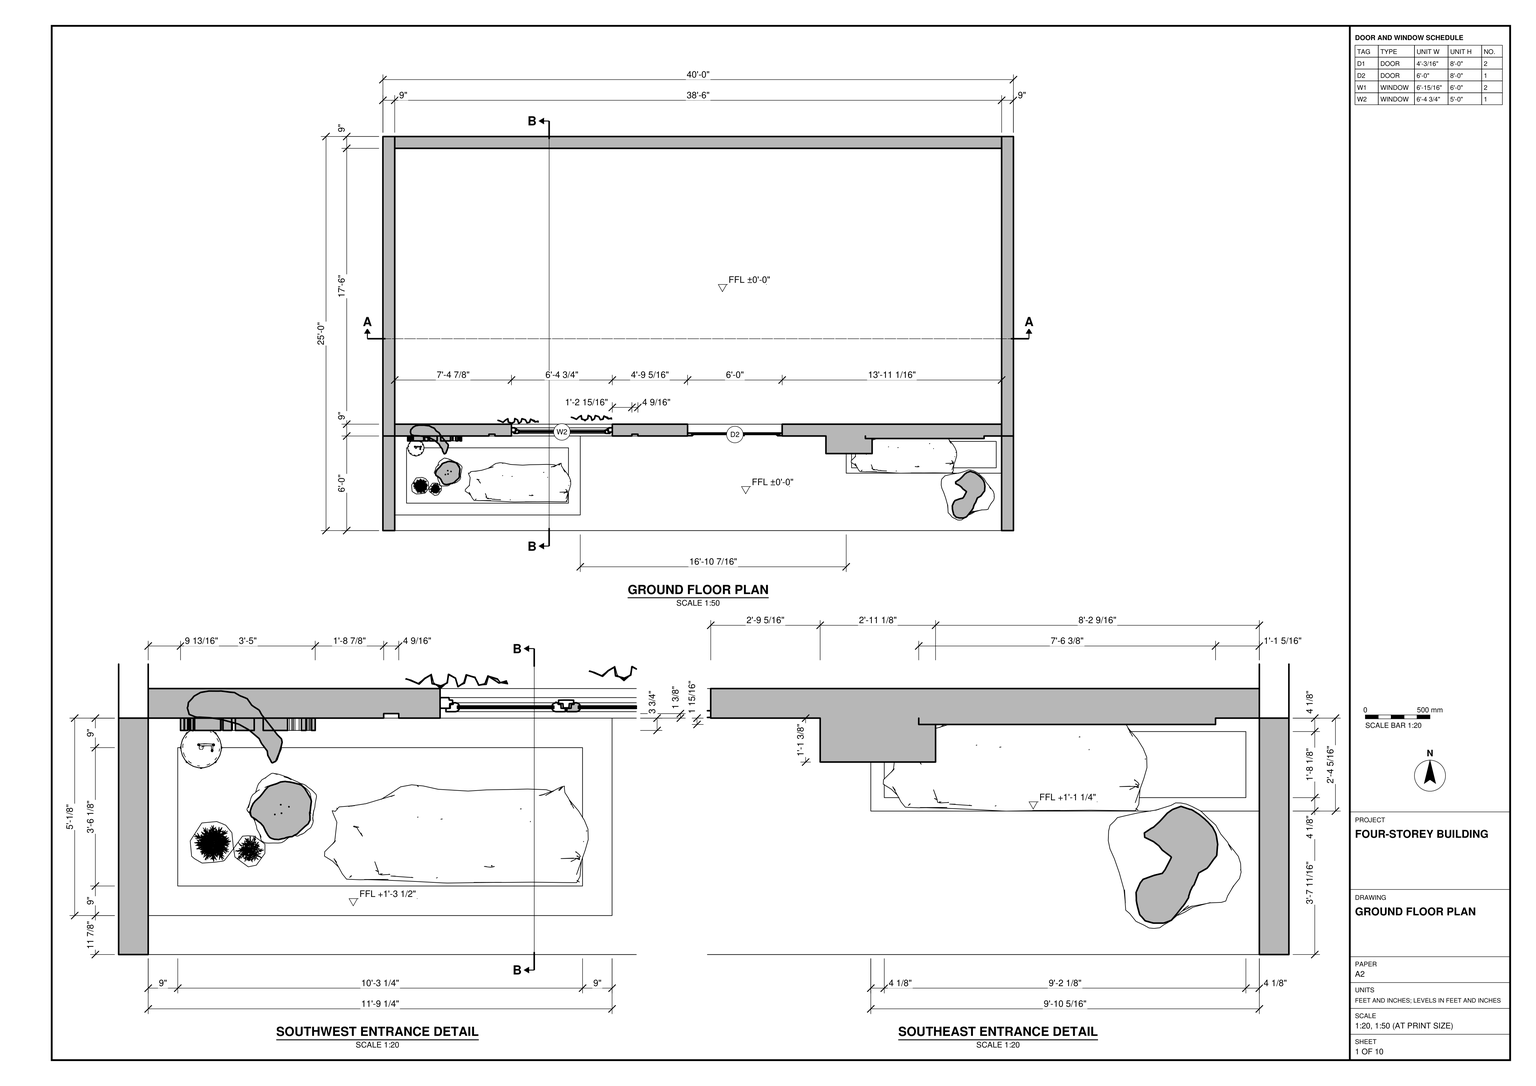
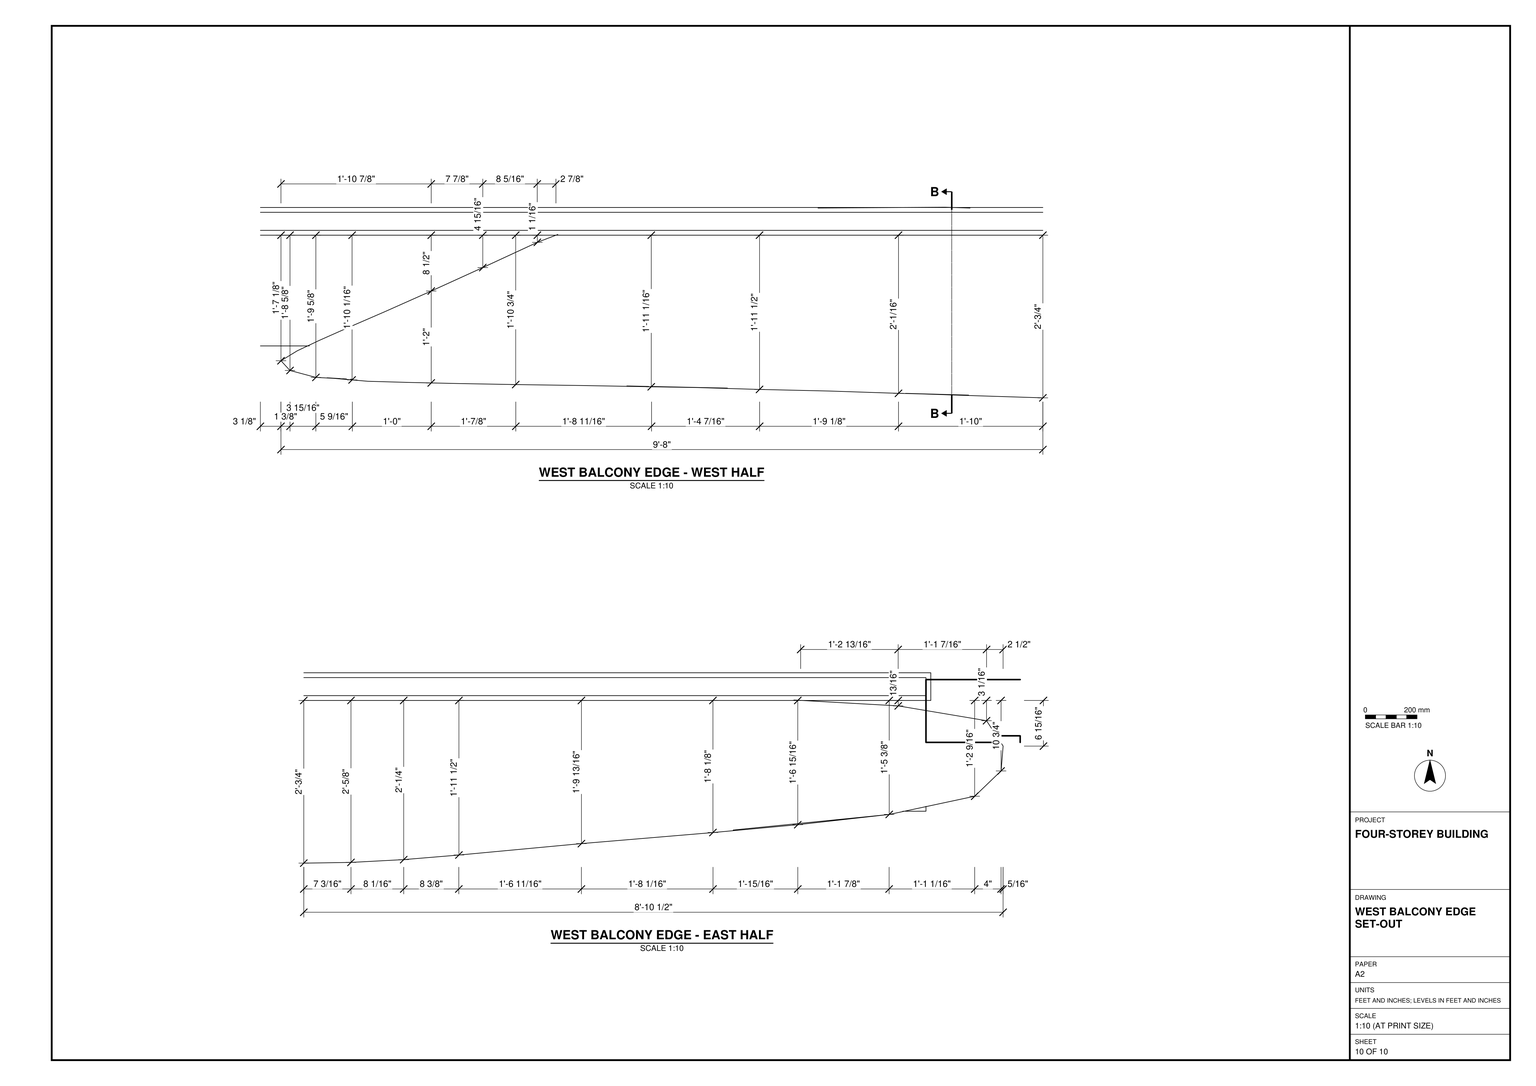
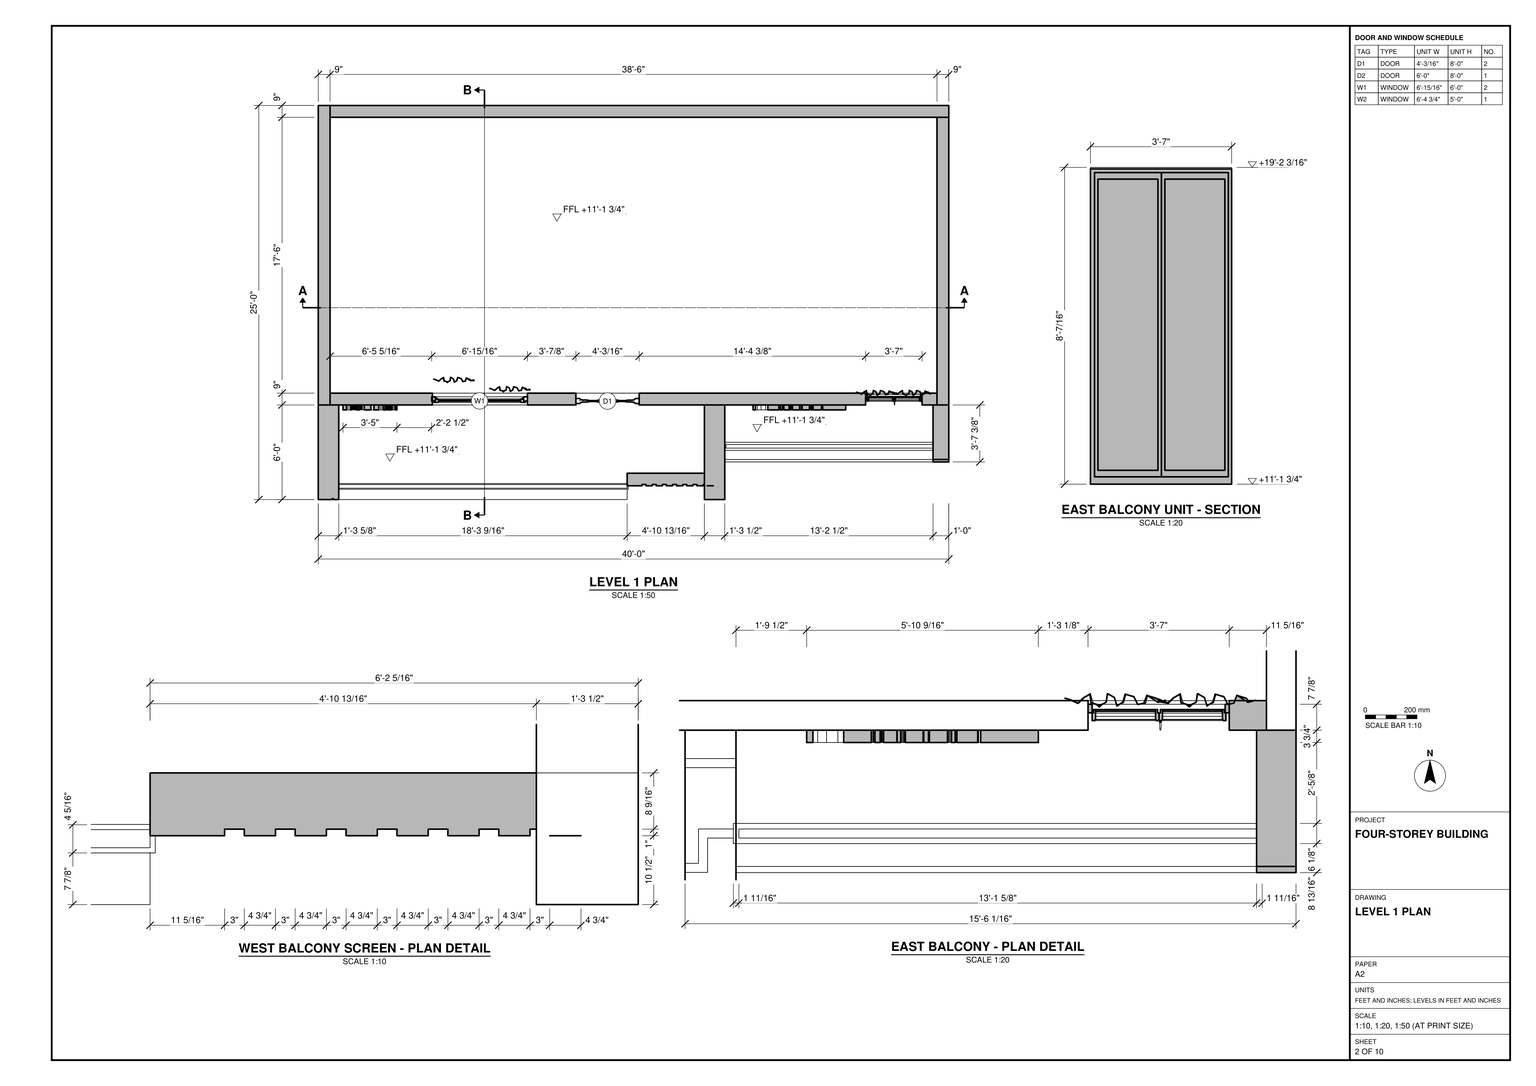
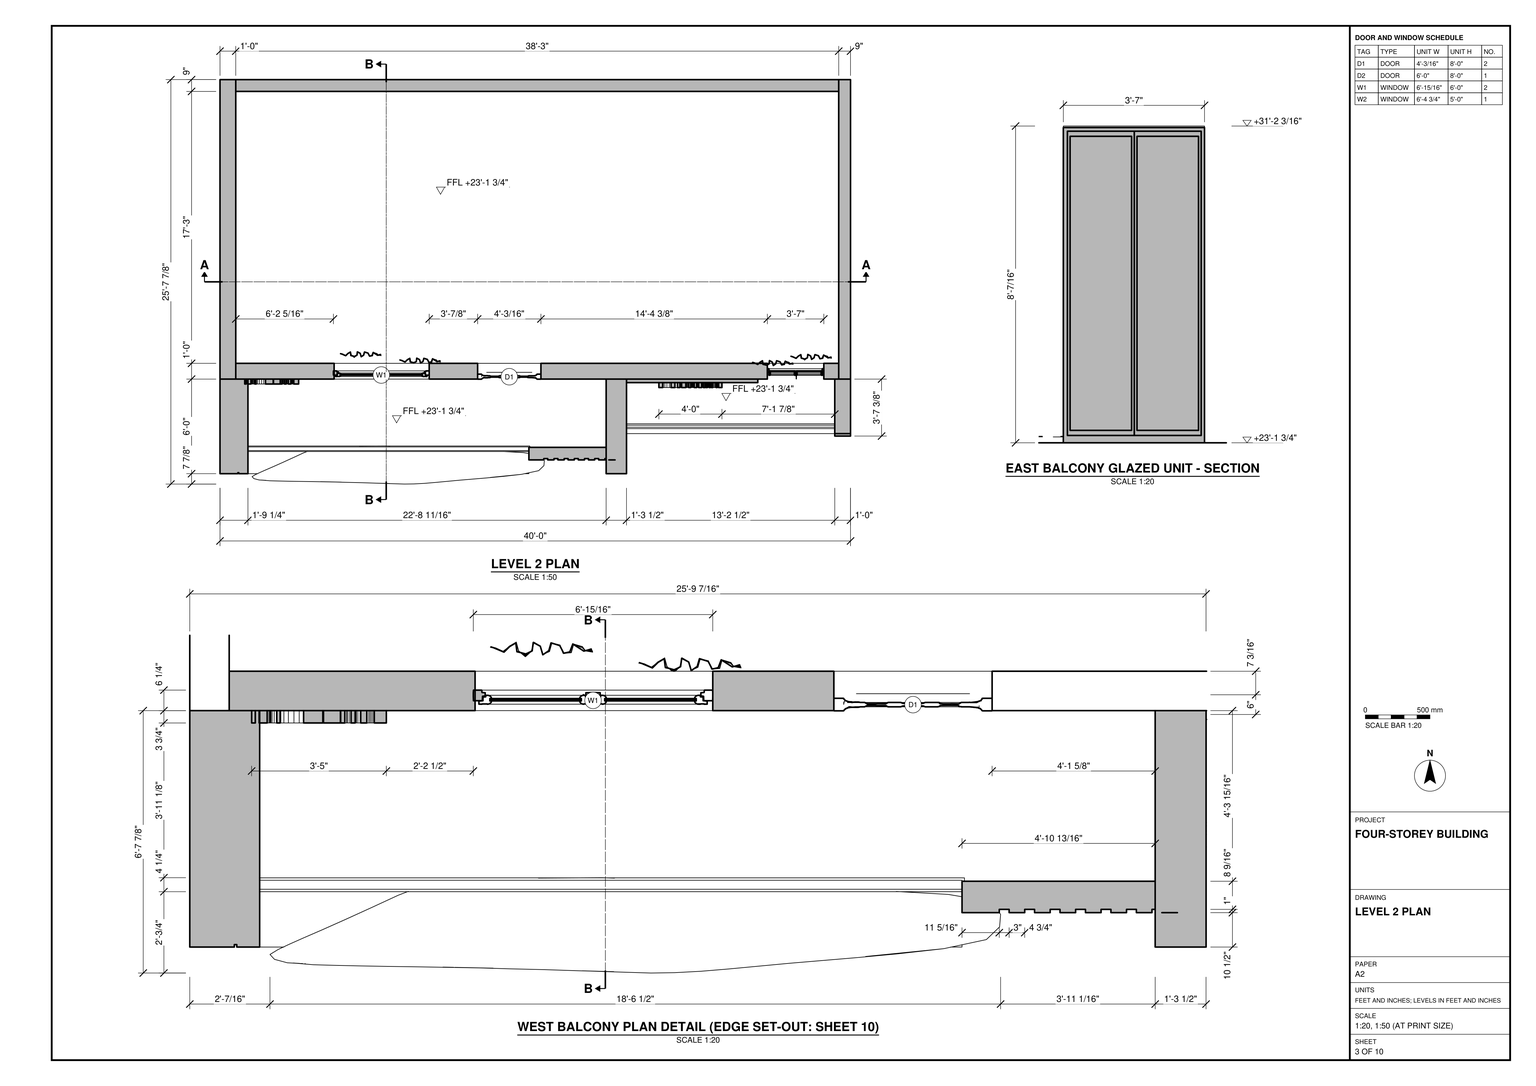
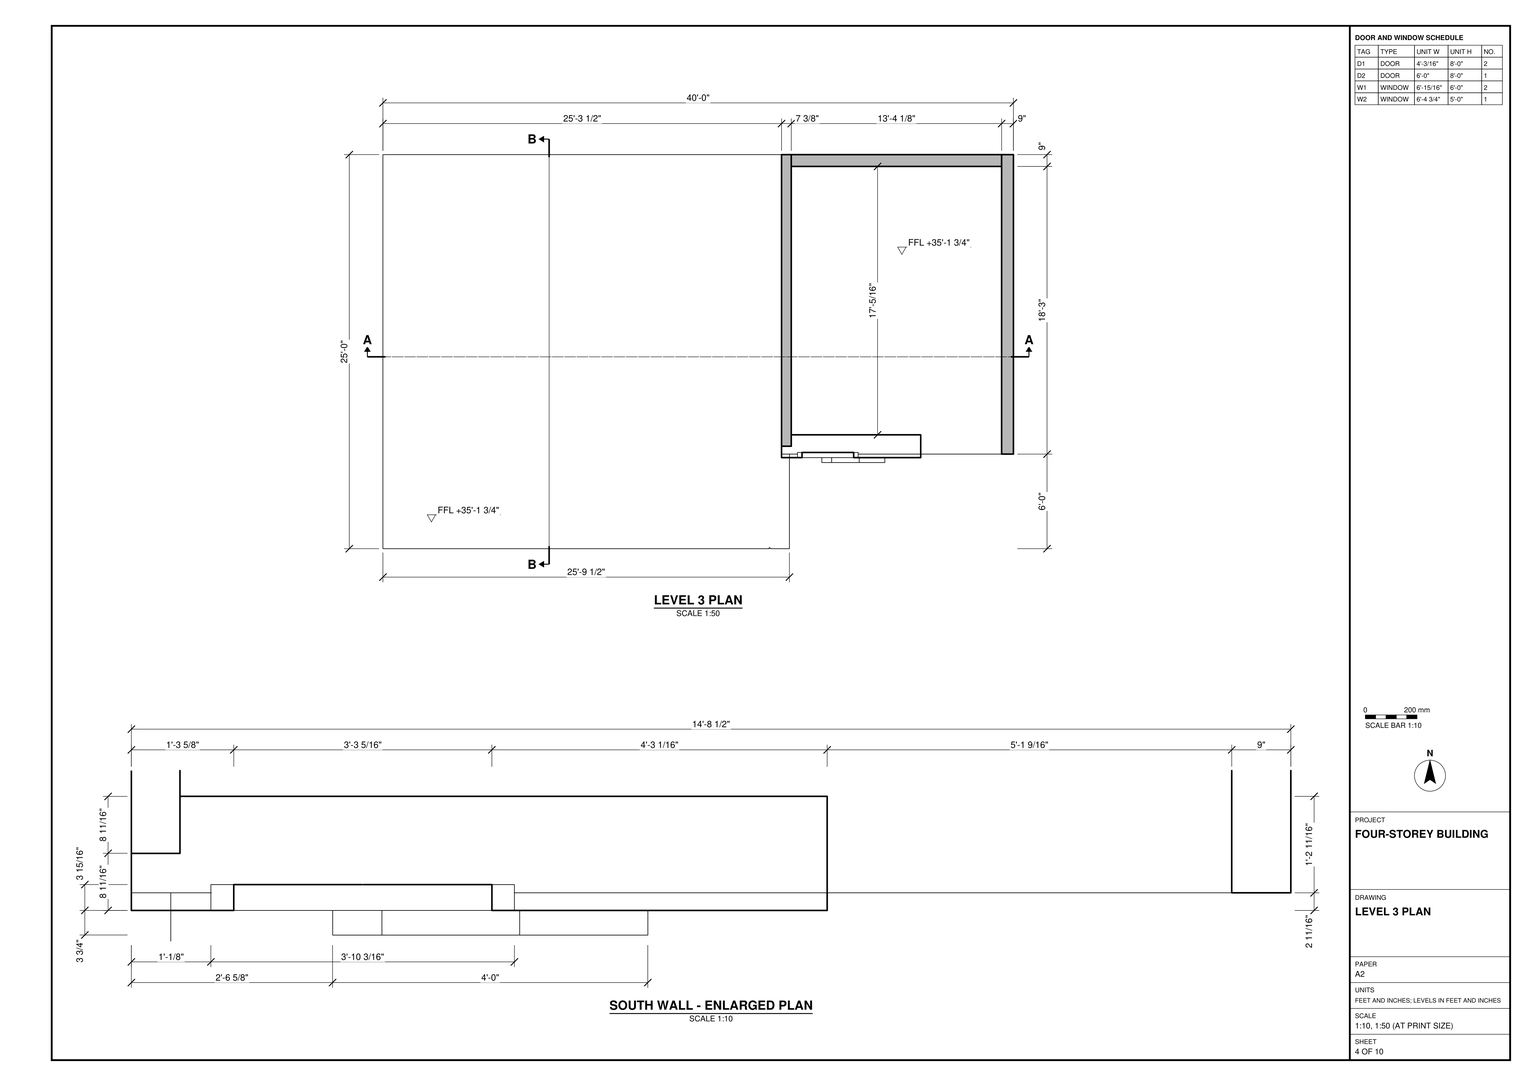
Build the four-storey building in SketchUp using task_files/diagram_01.pdf. Work in feet and inches. The overall model extents are 40'-0" from west to east, 25'-7 7/8" from front to back and 42'-7 3/4" in height. Set the floor levels to ±0'-0", +11'-1 3/4", +23'-1 3/4" and +35'-1 3/4".

Lay out the ground floor with the 9" walls shown in plan. Extend the side walls past the entrance wall to frame the 6'-0" deep entrance area. Place the front window west of the entrance door, and model the raised planting beds at the two ends of the entrance. Above it, distinguish the wider west balcony from the shallower east balcony. Use the enlarged details for the west balcony screen, the shaped balcony edge and the paired glazed panels at the east balcony.

Follow the plans, elevations and sections for the upper walls, floor slabs, openings and roof profile. Include stairs, built-in joinery and main furniture where shown. Keep walls, slabs, roof and each furniture or joinery piece in separate groups or components, and use components for repeated parts. Plants and other loose decorative items may be any suitable library components. Save one SketchUp model as output_files/four_storey_building_with_its_entrance_and_balconies.skp.

# SketchUp Ruby script. Lengths in inches.
U = 1.inch
M = Sketchup.active_model
def pt(a) = Geom::Point3d.new(a.map { |v| v * U })
def face(e, loops, mat)
  f = e.add_face(loops[0].map { |a| pt(a) })
  loops[1..].each { |l| e.add_face(l.map { |a| pt(a) }).erase! }
  f.material = f.back_material = mat if mat
  f
end
# faces: each face lists its corners as indices into pts; further lists are holes
def faces(e, pts, list, mat = nil) = list.each { |f| face(e, (f[0].is_a?(Array) ? f : [f]).map { |l| l.map { |i| pts[i] } }, mat) }
# xy, xz, yz: faces in a plane at the given z, y or x. An outline is a flat list of corners, or four numbers for a rectangle; further outlines are holes
def ring(l) = l.size == 4 ? [[l[0], l[1]], [l[2], l[1]], [l[2], l[3]], [l[0], l[3]]] : l.each_slice(2).to_a
def flat(e, list, mat, &to3) = list.each { |f| face(e, (f[0].is_a?(Array) ? f : [f]).map { |l| ring(l).map { |u, v| to3.(u, v) } }, mat) }
def xy(e, z, list, mat = nil) = flat(e, list, mat) { |x, y| [x, y, z] }
def xz(e, y, list, mat = nil) = flat(e, list, mat) { |x, z| [x, y, z] }
def yz(e, x, list, mat = nil) = flat(e, list, mat) { |y, z| [x, y, z] }
def lines(e, pts, list) = list.each { |a, b| e.add_line(pt(pts[a]), pt(pts[b])) }
# prism: a flat outline (further loops are holes) pulled along v
def prism(e, loops, v, mat = nil)
  f = face(e, loops, mat); d = Geom::Vector3d.new(v.map { |x| x * U })
  f.pushpull(f.normal.samedirection?(d) ? d.length : -d.length)
end
def box(e, o, s, mat = nil) = prism(e, [[o, [o[0] + s[0], o[1], o[2]], [o[0] + s[0], o[1] + s[1], o[2]], [o[0], o[1] + s[1], o[2]]]], [0, 0, s[2]], mat)
def at(x, y, z, deg = 0) = Geom::Transformation.translation(pt([x, y, z])) * Geom::Transformation.rotation(ORIGIN, Z_AXIS, deg.degrees)
def axes(o, x, y, z) = Geom::Transformation.new([*x, 0, *y, 0, *z, 0, *pt(o).to_a, 1])
def part(name) = M.definitions.add(name)
# library, detail: a bought-in or finely detailed component or shape, given as its bounding box
def library(name, o, s) = part(name).tap { |d| box(d.entities, o, s) }
def detail(e, o, s) = box(e.add_group.entities, o, s)
def put(e, d, t, mat = nil) = e.add_instance(d, t).tap { |i| i.material = mat if mat }
def group(e, t, mat = nil) = e.add_group.tap { |g| g.transformation = t; g.material = mat if mat }.entities
root = M.entities
M.materials.add("Emissive").color = [230, 236, 181]
M.materials.add("Marble White SSS 100cm").color = [222, 222, 222]
M.materials.add("[Color H07]").color = [0, 153, 153]
M.materials.add("[Translucent Glass Blue]").color = [100, 149, 237]
M.materials["[Translucent Glass Blue]"].alpha = 0.5
M.materials.add("[Wood Veneer 01]").color = [120, 70, 37]
c1 = library("Curtains 004",[-15.59,-2.26,0],[31.18,4.52,116.91])
c2 = library("Door 243 067",[-20.85,-3,0],[41.7,6,82.46])
c3 = library("Elegant door(double)",[38.88,29.07,0],[76.71,4.33,84.81])
c4 = library("porta_finestra_2ante",[2.73,-0.04,0],[81.59,5.98,96.46])
c5 = library("Window 46-15",[-34.06,-3.13,0],[68.12,6.24,59.06])
c6 = library("Viola hederacea 011",[-26.29,-11.24,-33.88],[55.62,29.03,38.84])
c7 = library("Viola hederacea 004",[-17.97,-14.58,0.39],[33.12,31.94,9.08])
c8 = library("False Aralia 002",[-20.33,-19.19,0],[40.48,38.23,49.87])
c9 = library("Potted Tree 19",[-18.04,-21.3125,0],[43.7,42.65,66.52])
c10 = library("Potted Plants 50-15",[-11.38,-6.89,0],[22.76,13.78,19.62])
c11 = library("Potted Plant 60-25",[-10.7,-10.47,0],[21.2,21.27,47.12])
c12 = library("Potted Flowers 111-27",[-6.96,-10.89,0.07],[14.96,24.75,20.38])
c13 = library("c103.dxf",[0,0,0],[4.7,1.18,0.06])
xy(root,-12,[[0,0,480,300]])
xy(root,0,[[0,0,9,72],[9,0,471,0,471,43.6875,352.6875,43.6875,352.6875,72,303.9375,72,303.9375,81,231.9375,81,231.9375,72,150.25,72,150.25,11.875,9,11.875],[471,0,480,72],[9,11.875,150.25,72],[0,72,9,300],
  [9,72,231.9375,81],[303.9375,72,471,81],[471,72,480,300],[9,81,471,291],[9,291,471,300]])
xy(root,8.19,[[367.29,70.0625,457.66,72]])
xy(root,10.875,[[17.99,20.87,141.26,63.01],[356.79,47.79,466.9,67.9]],"[Wood Veneer 01]")
xy(root,13.25,[[[352.6875,43.6875,471,72],[356.79,47.79,466.9,67.9]]],"[Wood Veneer 01]")
xy(root,15.5,[[[9,11.875,150.25,72],[17.99,20.87,141.26,63.01]]],"[Wood Veneer 01]")
xy(root,17.73,[[80.71,72,194.125,73.375]],"Emissive")
xy(root,22.3125,[[85.29,72,189.54,73.375]],"Emissive")
xy(root,36,[[97.875,72,174.625,81]],"Marble White SSS 100cm")
xy(root,39.07,[[337.27,58.625,346.66,72],[346.66,58.625,346.66,72,367.29,72,367.29,70.0625,372.41,70.0625,372.41,58.625]],"[Wood Veneer 01]")
xy(root,47.25,[[337.27,58.625,346.66,72],[346.66,58.625,372.41,58.625,372.41,70.0625,367.29,70.0625,367.29,72,346.66,72]],"[Wood Veneer 01]")
xy(root,69.27,[[337.27,58.625,346.66,72],[346.66,58.625,346.66,72,367.29,72,367.29,70.0625,372.41,70.0625,372.41,58.625]],"[Wood Veneer 01]")
xy(root,72,[[0,0,9,72],[471,0,480,72]])
xy(root,77.96,[[337.27,58.625,346.66,72],[346.66,58.625,372.41,58.625,372.41,70.0625,367.29,70.0625,367.29,72,346.66,72]],"[Wood Veneer 01]")
xy(root,96,[[231.9375,72,303.9375,81]])
xy(root,96,[[97.875,72,174.625,81]],"Marble White SSS 100cm")
xy(root,105.38,[[367.29,70.0625,457.66,72]],"Marble White SSS 100cm")
xy(root,108.8125,[[85.29,72,189.54,73.375]],"Emissive")
xy(root,113.4,[[80.71,72,194.125,73.375]],"Emissive")
xy(root,113.6875,[[293.96,0,309.47,72],[235.15,10.48,235.15,72,293.96,72,293.96,11.48,292.99,11.48,292.99,10.48,288.24,10.48,288.24,11.48,285.24,11.48,285.24,10.48,280.49,10.48,280.49,11.48,277.49,11.48,277.49,10.48,272.74,10.48,272.74,11.48,269.74,11.48,269.74,10.48,264.99,10.48,264.99,11.48,261.99,11.48,261.99,10.48,257.24,10.48,257.24,11.48,254.24,11.48,254.24,10.48,249.49,10.48,249.49,11.48,246.49,11.48,246.49,10.48]])
xy(root,117.6875,[[0,0,0,72,12.01,72,12.01,12.01,208.33,12.01,208.33,72,235.15,72,235.15,0]])
xy(root,118.875,[[[309.47,28.625,471,72],[318.44,37.6,462.02,63.02]],[471,28.625,480,72],[321.41,40.57,459.05,60.05]],"[Wood Veneer 01]")
xy(root,120,[[293.96,0,309.47,20.04],[[12.01,12.01,208.33,72],[19.9,19.9,200.44,64.11]],[293.96,20.04,309.47,72],[24.62,24.62,195.72,59.39],[471,30.5,480,72],
  [0,72,9,300],[9,72,471,81],[471,72,480,300],[9,81,471,291],[9,291,471,300]])
xy(root,120,[[309.47,30.5,471,72]],"[Wood Veneer 01]")
xy(root,120.3125,[[[318.44,37.6,462.02,63.02],[321.41,40.57,459.05,60.05]]])
xy(root,121.4375,[[[19.9,19.9,200.44,64.11],[24.62,24.62,195.72,59.39]]])
xy(root,128.5625,[[10.72,0,11.47,0.75],[11.47,0,235.15,0.75]])
xy(root,129.3125,[[11.47,0,235.15,0.75]])
xy(root,131.8125,[[309.47,28.625,468,30.5]],"[Wood Veneer 01]")
xy(root,133.75,[[15.6,0,235.15,8.65],[15.6,8.65,235.15,11.41],[15.6,11.41,235.15,11.41,235.15,20.04,309.47,20.04,309.47,30.5,468,30.5,468,39.15,310.35,39.15,310.35,41.91,468,41.91,468,72,459.66,72,459.66,81,416.67,81,416.67,72,244.3125,72,244.3125,81,196.125,81,196.125,72,15.6,72],[468,30.5,480,72],[310.35,39.15,468,41.91],
  [0,72,9,300],[9,72,196.125,81],[244.3125,72,416.67,81],[459.66,72,471,81],[471,72,480,291],
  [9,81,471,291],[9,291,480,300]])
xy(root,157.75,[[86.875,72,159.25,81]])
xy(root,169.75,[[15.6,8.65,235.15,11.41],[310.35,39.15,468,41.91]])
xy(root,169.75,[[[14.81,7.86,235.94,12.2],[15.6,8.65,235.15,11.41]],[[308.66,37.46,469.6875,43.6],[310.35,39.15,468,41.91]]],"[Color H07]")
xy(root,170.3125,[[[14.81,7.86,235.94,12.2],[15.6,8.65,235.15,11.41]],[15.6,8.65,235.15,11.41],[[308.66,37.46,469.6875,43.6],[310.35,39.15,468,41.91]],[310.35,39.15,468,41.91]],"[Color H07]")
xy(root,181.75,[[0,0,10.72,0,10.72,0.75,11.47,0.75,11.47,0,15.6,0,15.6,72,0,72]])
xy(root,229.75,[[86.875,72,159.25,81],[196.125,72,244.3125,81],[416.67,72,459.66,81]])
xy(root,253.75,[[0,0,0,72,21.28,72,21.28,0,14.3125,0,14.3125,0.75,13.5625,0.75,13.5625,0],[0,72,9,300],[9,72,471,81],[471,72,480,291],[9,81,471,291],
  [9,291,480,300]])
xy(root,253.75,[[[21.28,0,21.28,72,480,72,480,30.5,309.47,30.5,309.47,20.04,235.15,20.04,235.15,0],[31.97,10.6875,224.46,61.3125],[322.45,41.96,453.17,60.54]],[35.875,14.6,220.55,57.4],[325.58,45.1,450.03,57.4]],"[Wood Veneer 01]")
xy(root,255.1875,[[[31.97,10.6875,224.46,61.3125],[35.875,14.6,220.55,57.4]],[[322.45,41.96,453.17,60.54],[325.58,45.1,450.03,57.4]]],"[Wood Veneer 01]")
xy(root,256.43,[[21.28,0,235.15,0.75]],"[Wood Veneer 01]")
xy(root,257.18,[[21.28,0,235.15,0.75]],"[Wood Veneer 01]")
xy(root,259.86,[[21.28,0,235.15,0.75]],"[Wood Veneer 01]")
xy(root,260.61,[[21.28,0,235.15,0.75]],"[Wood Veneer 01]")
xy(root,263.29,[[21.28,0,235.15,0.75]],"[Wood Veneer 01]")
xy(root,264.04,[[21.28,0,235.15,0.75]],"[Wood Veneer 01]")
xy(root,266.71,[[21.28,0,235.15,0.75]],"[Wood Veneer 01]")
xy(root,267.46,[[21.28,0,235.15,0.75]],"[Wood Veneer 01]")
xy(root,270.14,[[21.28,0,235.15,0.75]],"[Wood Veneer 01]")
xy(root,270.89,[[21.28,0,235.15,0.75]],"[Wood Veneer 01]")
xy(root,273.57,[[21.28,0,235.15,0.75]],"[Wood Veneer 01]")
xy(root,274.32,[[21.28,0,235.15,0.75]],"[Wood Veneer 01]")
xy(root,277.75,[[21.28,17.6,235.15,20.35],[235.15,20.04,309.47,20.04,309.47,72,244.3125,72,244.3125,84,196.125,84,196.125,72,21.28,72,21.28,20.35,235.15,20.35],[309.47,30.5,480,30.5,480,72,459.66,72,459.66,84,416.67,84,416.67,72,409.41,72,409.41,69.3125,309.47,69.3125,309.47,36.9,468,36.9,468,35.36,309.47,35.36],[309.47,35.36,314.32,36.9],[314.32,35.36,468,36.9],
  [0,72,12,300],[12,72,196.125,84],[244.3125,72,416.67,84],[459.66,72,471,84],[471,72,480,300],
  [12,84,471,291],[12,291,471,300]])
xy(root,277.75,[[21.28,0,235.15,17.6]],"[Wood Veneer 01]")
xy(root,301.75,[[86.875,72,159.25,84]])
xy(root,313.75,[[21.28,17.6,235.15,20.35],[309.47,35.36,468,36.9]])
xy(root,313.75,[[[20.54,16.86,235.89,21.08],[21.28,17.6,235.15,20.35]],[[308.41,34.3,469.06,37.96],[309.47,35.36,468,36.9]]],"[Color H07]")
xy(root,314.3125,[[[20.54,16.86,235.89,21.08],[21.28,17.6,235.15,20.35]],[21.28,17.6,235.15,20.35],[[308.41,34.3,469.06,37.96],[309.47,35.36,468,36.9]],[309.47,35.36,468,36.9]],"[Color H07]")
xy(root,337.75,[[468,28.625,480,30.5],[468,30.5,480,72]])
xy(root,373.75,[[86.875,72,159.25,84],[196.125,72,244.3125,84],[416.67,72,459.66,84]])
xy(root,397.75,[[0,0,12,72],[[21.28,0,21.28,72,293.96,72,293.96,20.04,235.15,20.04,235.15,10.48,246.49,10.48,246.49,11.48,249.49,11.48,249.49,10.48,254.24,10.48,254.24,11.48,257.24,11.48,257.24,10.48,261.99,10.48,261.99,11.48,264.99,11.48,264.99,10.48,269.74,10.48,269.74,11.48,272.74,11.48,272.74,10.48,277.49,10.48,277.49,11.48,280.49,11.48,280.49,10.48,285.24,10.48,285.24,11.48,288.24,11.48,288.24,10.48,292.99,10.48,292.99,11.48,293.96,11.48,293.96,0],[155.72,13.26,230.91,13.26,230.91,69.88,223.53,69.88,223.53,20.57,162.28,20.57,162.28,69.88,155.72,69.88],[40.85,13.44,116.03,13.44,116.03,70.07,108.66,70.07,108.66,20.76,47.41,20.76,47.41,70.07,40.85,70.07]],[293.96,0,309.47,72],[235.15,10.48,246.49,10.48,246.49,11.48,249.49,11.48,249.49,10.48,254.24,10.48,254.24,11.48,257.24,11.48,257.24,10.48,261.99,10.48,261.99,11.48,264.99,11.48,264.99,10.48,269.74,10.48,269.74,11.48,272.74,11.48,272.74,10.48,277.49,10.48,277.49,11.48,280.49,11.48,280.49,10.48,285.24,10.48,285.24,11.48,288.24,11.48,288.24,10.48,292.99,10.48,292.99,11.48,293.96,11.48,293.96,20.04,235.15,20.04],[0,72,12,300],
  [12,84,471,291],[12,291,471,300]])
xy(root,399.9375,[[155.72,13.26,155.72,69.88,162.28,69.88,162.28,20.57,223.53,20.57,223.53,69.88,230.91,69.88,230.91,13.26],[40.85,13.44,40.85,70.07,47.41,70.07,47.41,20.76,108.66,20.76,108.66,70.07,116.03,70.07,116.03,13.44]])
xy(root,403,[[14.3125,0,293.96,0.75],[293.96,0,294.71,0.75]])
xy(root,403.75,[[13.5625,0,293.96,0.75]])
xy(root,421.75,[[0,0,293.96,0,293.96,0.75,294.71,0.75,294.71,0,309.47,0,309.47,69.3125,303.47,69.3125,303.47,300,0,300],[303.47,69.3125,309.47,72],[303.47,72,303.47,78,310.87,78,310.87,86.6875,409.41,86.6875,409.41,72],[409.41,72,471,72,471,291,310.87,291,310.87,86.6875,409.41,86.6875],[471,72,480,300],
  [303.47,78,310.87,300],[310.87,291,471,300]])
xy(root,493.75,[[292.53,57.5625,292.53,300,303.47,300,303.47,69.3125,409.41,69.3125,409.41,78,471,78,471,72,480,72,480,57.5625],[303.47,69.3125,310.87,72],[310.87,69.3125,409.41,72],[303.47,72,310.87,78],[310.87,72,409.41,78],
  [471,72,480,300],[303.47,78,310.87,300],[310.87,78,409.41,86.6875],[310.87,291,471,300]])
xy(root,499.75,[[[292.53,57.5625,480,300],[310.87,78,471,291]]])
xz(root,0,[[0,-12,480,0],[0,0,9,72],[471,0,480,72],[293.96,113.6875,309.47,120],[0,117.6875,235.15,117.6875,235.15,128.5625,10.72,128.5625,10.72,181.75,0,181.75],
  [293.96,120,309.47,397.75],[11.47,129.3125,235.15,129.3125,235.15,133.75,15.6,133.75,15.6,181.75,11.47,181.75],[0,253.75,13.5625,397.75],[14.3125,253.75,21.28,397.75],[0,397.75,13.5625,397.75,13.5625,403.75,293.96,403.75,293.96,421.75,0,421.75],
  [14.3125,397.75,309.47,397.75,309.47,421.75,294.71,421.75,294.71,403,14.3125,403]])
xz(root,0,[[21.28,253.75,235.15,256.43],[21.28,257.18,235.15,259.86],[21.28,260.61,235.15,263.29],[21.28,264.04,235.15,266.71],[21.28,267.46,235.15,270.14],
  [21.28,270.89,235.15,273.57],[21.28,274.32,235.15,277.75]],"[Wood Veneer 01]")
xz(root,0.75,[[10.72,128.5625,235.15,128.5625,235.15,129.3125,11.47,129.3125,11.47,181.75,10.72,181.75],[13.5625,253.75,14.3125,397.75],[13.5625,397.75,14.3125,403],[13.5625,403,294.71,403,294.71,421.75,293.96,421.75,293.96,403.75,13.5625,403.75]])
xz(root,0.75,[[21.28,256.43,235.15,257.18],[21.28,259.86,235.15,260.61],[21.28,263.29,235.15,264.04],[21.28,266.71,235.15,267.46],[21.28,270.14,235.15,270.89],
  [21.28,273.57,235.15,274.32]],"[Wood Veneer 01]")
xz(root,7.86,[[14.81,169.75,235.94,170.3125]],"[Color H07]")
xz(root,8.65,[[15.6,169.75,235.15,170.3125]])
xz(root,8.65,[[15.6,133.75,235.15,169.75]],"[Translucent Glass Blue]")
xz(root,10.48,[[235.15,113.6875,241.74,397.75],[241.74,113.6875,246.49,397.75],[249.49,113.6875,254.24,397.75],[257.24,113.6875,261.99,397.75],[264.99,113.6875,269.74,397.75],
  [272.74,113.6875,277.49,397.75],[280.49,113.6875,285.24,397.75],[288.24,113.6875,292.99,397.75],[295.99,113.6875,300.74,397.75]])
xz(root,10.6875,[[31.97,253.75,224.46,255.1875]],"Emissive")
xz(root,11.41,[[226.5,133.75,235.15,169.75],[15.6,169.75,226.5,170.3125],[226.5,169.75,235.15,170.3125]])
xz(root,11.41,[[15.6,133.75,226.5,169.75]],"[Translucent Glass Blue]")
xz(root,11.48,[[246.49,113.6875,249.49,397.75],[254.24,113.6875,257.24,397.75],[261.99,113.6875,264.99,397.75],[269.74,113.6875,272.74,397.75],[277.49,113.6875,280.49,397.75],
  [285.24,113.6875,288.24,397.75],[292.99,113.6875,293.96,397.75]])
xz(root,11.875,[[9,0,150.25,15.5]],"[Wood Veneer 01]")
xz(root,12.01,[[12.01,117.6875,208.33,120]])
xz(root,12.2,[[226.5,169.75,235.94,170.3125]])
xz(root,12.2,[[14.81,169.75,226.5,170.3125]],"[Color H07]")
xz(root,13.26,[[155.72,397.75,230.91,399.9375]],"Emissive")
xz(root,13.44,[[40.85,397.75,116.03,399.9375]],"Emissive")
xz(root,14.6,[[35.875,253.75,220.55,255.1875]],"Emissive")
xz(root,16.86,[[20.54,313.75,235.89,314.3125]],"[Color H07]")
xz(root,17.6,[[21.28,313.75,235.15,314.3125]])
xz(root,17.6,[[21.28,277.75,235.15,313.75]],"[Translucent Glass Blue]")
xz(root,19.9,[[19.9,120,200.44,121.4375]],"Emissive")
xz(root,20.04,[[293.96,120,309.47,133.75],[235.15,133.75,293.96,253.75],[293.96,253.75,309.47,277.75],[235.15,277.75,293.96,397.75]])
xz(root,20.35,[[21.28,313.75,235.15,314.3125]])
xz(root,20.35,[[21.28,277.75,235.15,313.75]],"[Translucent Glass Blue]")
xz(root,20.57,[[162.28,397.75,223.53,399.9375]],"Emissive")
xz(root,20.76,[[47.41,397.75,108.66,399.9375]],"Emissive")
xz(root,20.87,[[17.99,10.875,141.26,15.5]],"[Wood Veneer 01]")
xz(root,21.08,[[20.54,313.75,235.89,314.3125]],"[Color H07]")
xz(root,24.62,[[24.62,120,195.72,121.4375]],"Emissive")
xz(root,28.625,[[309.47,118.875,480,118.875,480,337.75,468,337.75,468,131.8125,309.47,131.8125]],"[Wood Veneer 01]")
xz(root,30.5,[[309.47,120,309.47,131.8125,468,131.8125,468,133.75,480,133.75,480,120],[309.47,131.8125,468,133.75],[468,133.75,480,253.75],[309.47,253.75,468,277.75],[468,253.75,480,277.75],
  [468,277.75,480,337.75]])
xz(root,34.3,[[308.41,313.75,314.32,314.3125]])
xz(root,34.3,[[314.32,313.75,469.06,314.3125]],"[Color H07]")
xz(root,35.36,[[309.47,313.75,314.32,314.3125],[314.32,313.75,468,314.3125]])
xz(root,35.36,[[309.47,277.75,314.32,313.75],[314.32,277.75,468,313.75]],"[Translucent Glass Blue]")
xz(root,36.9,[[309.47,277.75,314.32,313.75],[309.47,313.75,314.32,314.3125],[314.32,313.75,468,314.3125]])
xz(root,36.9,[[314.32,277.75,468,313.75]],"[Translucent Glass Blue]")
xz(root,37.46,[[308.66,169.75,469.6875,170.3125]],"[Color H07]")
xz(root,37.6,[[318.44,118.875,462.02,120.3125]],"Emissive")
xz(root,37.96,[[308.41,313.75,314.32,314.3125]])
xz(root,37.96,[[314.32,313.75,469.06,314.3125]],"[Color H07]")
xz(root,39.15,[[310.35,169.75,468,170.3125]])
xz(root,39.15,[[310.35,133.75,468,169.75]],"[Translucent Glass Blue]")
xz(root,40.57,[[321.41,118.875,459.05,120.3125]],"Emissive")
xz(root,41.91,[[310.35,169.75,468,170.3125]])
xz(root,41.91,[[310.35,133.75,468,169.75]],"[Translucent Glass Blue]")
xz(root,41.96,[[322.45,253.75,453.17,255.1875]],"Emissive")
xz(root,43.6,[[308.66,169.75,469.6875,170.3125]],"[Color H07]")
xz(root,43.6875,[[352.6875,0,471,13.25]],"[Wood Veneer 01]")
xz(root,45.1,[[325.58,253.75,450.03,255.1875]],"Emissive")
xz(root,47.79,[[356.79,10.875,466.9,13.25]],"[Wood Veneer 01]")
xz(root,57.4,[[35.875,253.75,220.55,255.1875]])
xz(root,57.4,[[325.58,253.75,450.03,255.1875]],"Emissive")
xz(root,57.5625,[[292.53,493.75,480,499.75]])
xz(root,58.625,[[337.27,39.07,346.66,47.25],[346.66,39.07,372.41,47.25],[337.27,69.27,346.66,77.96],[346.66,69.27,372.41,77.96]],"[Wood Veneer 01]")
xz(root,59.39,[[24.62,120,195.72,121.4375]])
xz(root,60.05,[[321.41,118.875,459.05,120.3125]],"Emissive")
xz(root,60.54,[[322.45,253.75,453.17,255.1875]],"Emissive")
xz(root,61.3125,[[31.97,253.75,224.46,255.1875]],"Emissive")
xz(root,63.01,[[17.99,10.875,141.26,15.5]],"[Wood Veneer 01]")
xz(root,63.02,[[318.44,118.875,462.02,120.3125]],"Emissive")
xz(root,64.11,[[19.9,120,200.44,121.4375]],"Emissive")
xz(root,67.9,[[457.66,10.875,466.9,13.25]])
xz(root,67.9,[[356.79,10.875,367.29,13.25],[367.29,10.875,457.66,13.25]],"[Wood Veneer 01]")
xz(root,69.3125,[[[309.47,277.75,409.41,277.75,409.41,493.75,303.47,493.75,303.47,421.75,309.47,421.75],[340.62,433.9,334.57,434.18,328.81,436.03,323.71,439.3,319.64,443.77,316.86,449.15,315.58,455.07,315.86,461.11,317.7,466.88,320.97,471.97,325.45,476.05,330.83,478.82,336.74,480.11,342.79,479.83,348.56,477.98,353.65,474.71,357.72,470.24,360.5,464.86,361.79,458.94,361.5,452.9,359.66,447.13,356.39,442.04,351.91,437.96,346.53,435.1875]]])
xz(root,69.88,[[155.72,397.75,162.28,399.9375],[223.53,397.75,230.91,399.9375]],"Emissive")
xz(root,70.0625,[[367.29,39.07,372.41,47.25],[367.29,69.27,372.41,77.96]])
xz(root,70.0625,[[367.29,8.19,457.66,8.19,457.66,105.38,367.29,105.38,367.29,77.96,372.41,77.96,372.41,69.27,367.29,69.27,367.29,47.25,372.41,47.25,372.41,39.07,367.29,39.07]],"Marble White SSS 100cm")
xz(root,70.07,[[40.85,397.75,47.41,399.9375],[108.66,397.75,116.03,399.9375]],"Emissive")
xz(root,72,[[0,0,9,72],[9,0,150.25,15.5],[352.6875,0,471,0,471,13.25,457.66,13.25,457.66,8.19,367.29,8.19,367.29,13.25,352.6875,13.25],[471,0,480,72],[367.29,8.19,457.66,13.25],
  [337.27,69.27,346.66,77.96],[346.66,69.27,367.29,77.96],[0,72,9,117.6875],[471,72,480,118.875],[0,117.6875,9,120],
  [9,117.6875,12.01,120],[208.33,117.6875,293.96,120],[293.96,120,309.47,133.75],[0,133.75,9,181.75],[9,133.75,15.6,181.75],
  [[15.6,133.75,196.125,133.75,196.125,229.75,244.3125,229.75,244.3125,133.75,293.96,133.75,293.96,253.75,9,253.75,9,181.75,15.6,181.75],[86.875,157.75,159.25,229.75]],[293.96,133.75,309.47,253.75],[309.47,133.75,416.67,133.75,416.67,229.75,459.66,229.75,459.66,133.75,468,133.75,468,253.75,309.47,253.75],[468,133.75,471,253.75],[471,133.75,480,253.75],
  [0,181.75,9,253.75],[293.96,253.75,309.47,277.75],[468,253.75,471,277.75],[471,253.75,480,277.75],[0,277.75,12,397.75],
  [12,277.75,21.28,397.75],[[21.28,277.75,196.125,277.75,196.125,373.75,244.3125,373.75,244.3125,277.75,293.96,277.75,293.96,397.75,21.28,397.75],[86.875,301.75,159.25,373.75]],[293.96,277.75,309.47,397.75],[309.47,277.75,409.41,421.75],[409.41,277.75,416.67,277.75,416.67,373.75,459.66,373.75,459.66,277.75,468,277.75,468,337.75,471,337.75,471,421.75,409.41,421.75],
  [468,277.75,471,337.75],[471,277.75,480,337.75],[471,337.75,480,421.75],[471,421.75,480,493.75]])
xz(root,72,[[[150.25,0,231.9375,0,231.9375,96,303.9375,96,303.9375,0,346.66,0,346.66,39.07,337.27,39.07,337.27,47.25,346.66,47.25,346.66,69.27,337.27,69.27,337.27,77.96,346.66,77.96,346.66,118.875,309.47,118.875,309.47,113.6875,235.15,113.6875,235.15,117.6875,208.33,117.6875,208.33,120,12.01,120,12.01,117.6875,9,117.6875,9,15.5,150.25,15.5],[80.71,17.73,194.125,113.4]],[[85.29,22.3125,189.54,108.8125],[97.875,36,174.625,96]]],"Marble White SSS 100cm")
xz(root,72,[[346.66,0,352.6875,0,352.6875,13.25,367.29,13.25,367.29,39.07,346.66,39.07],[457.66,13.25,471,13.25,471,118.875,346.66,118.875,346.66,77.96,367.29,77.96,367.29,105.38,457.66,105.38],[346.66,47.25,367.29,69.27]],"[Wood Veneer 01]")
xz(root,73.25,[[[340.62,433.9,346.53,435.1875,351.91,437.96,356.39,442.04,359.66,447.13,361.5,452.9,361.79,458.94,360.5,464.86,357.72,470.24,353.65,474.71,348.56,477.98,342.79,479.83,336.74,480.11,330.83,478.82,325.45,476.05,320.97,471.97,317.7,466.88,315.86,461.11,315.58,455.07,316.86,449.15,319.64,443.77,323.71,439.3,328.81,436.03,334.57,434.18],[338.68,445,335.58,445.41,332.68,446.61,330.2,448.52,328.29,451,327.09,453.9,326.68,457,327.09,460.11,328.29,463,330.2,465.49,332.68,467.4,335.58,468.6,338.68,469,341.79,468.6,344.68,467.4,347.17,465.49,349.07,463,350.27,460.11,350.68,457,350.27,453.9,349.07,451,347.17,448.52,344.68,446.61,341.79,445.41]]])
xz(root,73.375,[[[80.71,17.73,194.125,113.4],[85.29,22.3125,189.54,108.8125]]],"Marble White SSS 100cm")
xz(root,78,[[303.47,421.75,310.87,493.75],[310.87,493.75,471,499.75]])
xz(root,81,[[[9,0,9,120,471,120,471,0,303.9375,0,303.9375,96,231.9375,96,231.9375,0],[97.875,36,174.625,96]],[[9,133.75,9,253.75,471,253.75,471,133.75,459.66,133.75,459.66,229.75,416.67,229.75,416.67,133.75,244.3125,133.75,244.3125,229.75,196.125,229.75,196.125,133.75],[86.875,157.75,159.25,229.75]]])
xz(root,84,[[[12,277.75,12,397.75,471,397.75,471,277.75,459.66,277.75,459.66,373.75,416.67,373.75,416.67,277.75,244.3125,277.75,244.3125,373.75,196.125,373.75,196.125,277.75],[86.875,301.75,159.25,373.75]]])
xz(root,86.6875,[[[310.87,421.75,409.41,493.75],[342.5,441.49,346,442.04,349.23,443.48,351.98,445.71,354.0625,448.57,355.33,451.88,355.7,455.4,355.15,458.9,353.71,462.13,351.48,464.88,348.61,466.96,345.31,468.23,341.79,468.6,338.29,468.04,335.06,466.6,332.31,464.37,330.23,461.51,328.96,458.2,328.59,454.68,329.15,451.1875,330.59,447.95,332.81,445.2,335.68,443.12,338.98,441.85]]])
xz(root,291,[[9,0,471,120],[9,133.75,471,253.75],[471,133.75,480,253.75],[12,277.75,471,397.75],[310.87,421.75,471,493.75],
  [310.87,493.75,471,499.75]])
xz(root,300,[[0,-12,480,0],[0,0,9,120],[9,0,471,120],[471,0,480,120],[0,120,480,133.75],
  [0,133.75,9,253.75],[9,133.75,480,253.75],[0,253.75,480,277.75],[0,277.75,12,397.75],[12,277.75,471,397.75],
  [471,277.75,480,397.75],[0,397.75,480,421.75],[303.47,421.75,310.87,493.75],[310.87,421.75,471,493.75],[471,421.75,480,493.75],
  [292.53,493.75,480,499.75]])
yz(root,0,[[0,-12,300,0],[0,0,72,72],[72,0,300,120],[0,117.6875,0,133.75,300,133.75,300,120,72,120,72,117.6875],[0,133.75,72,181.75],
  [72,133.75,300,253.75],[0,253.75,300,277.75],[0,277.75,72,397.75],[72,277.75,300,397.75],[0,397.75,300,421.75]])
yz(root,9,[[0,0,11.875,0,11.875,15.5,72,15.5,72,72,0,72],[11.875,0,72,15.5],[72,0,81,120],[81,0,291,120],[291,0,300,120],
  [72,133.75,81,253.75],[81,133.75,291,253.75],[291,133.75,300,253.75]])
yz(root,10.72,[[0,128.5625,0.75,181.75]])
yz(root,11.47,[[0,129.3125,0.75,181.75]])
yz(root,12,[[72,277.75,84,397.75],[84,277.75,291,397.75],[291,277.75,300,397.75]])
yz(root,12.01,[[12.01,117.6875,72,120]])
yz(root,13.5625,[[0,253.75,0.75,397.75],[0,397.75,0.75,403],[0,403,0.75,403.75]])
yz(root,14.3125,[[0,253.75,0.75,397.75],[0,397.75,0.75,403]])
yz(root,14.81,[[7.86,169.75,12.2,170.3125]])
yz(root,15.6,[[0,133.75,8.65,133.75,8.65,170.3125,11.41,170.3125,11.41,133.75,72,133.75,72,181.75,0,181.75],[8.65,133.75,11.41,169.75],[8.65,169.75,11.41,170.3125]])
yz(root,17.99,[[20.87,10.875,63.01,15.5]],"[Wood Veneer 01]")
yz(root,19.9,[[19.9,120,64.11,121.4375]],"Emissive")
yz(root,20.54,[[16.86,313.75,21.08,314.3125]])
yz(root,21.28,[[0,277.75,17.6,277.75,17.6,314.3125,20.35,314.3125,20.35,277.75,72,277.75,72,397.75,0,397.75],[17.6,277.75,20.35,313.75],[17.6,313.75,20.35,314.3125]])
yz(root,21.28,[[0,256.43,0.75,257.18],[0,259.86,0.75,260.61],[0,263.29,0.75,264.04],[0,266.71,0.75,267.46],[0,270.14,0.75,270.89],
  [0,273.57,0.75,274.32]],"[Wood Veneer 01]")
yz(root,24.62,[[24.62,120,59.39,121.4375]],"Emissive")
yz(root,31.97,[[10.6875,253.75,61.3125,255.1875]],"Emissive")
yz(root,35.875,[[14.6,253.75,57.4,255.1875]],"Emissive")
yz(root,40.85,[[13.44,397.75,70.07,399.9375]],"Emissive")
yz(root,47.41,[[20.76,397.75,70.07,399.9375]],"Emissive")
yz(root,80.71,[[72,17.73,73.375,113.4]],"Emissive")
yz(root,85.29,[[72,22.3125,73.375,108.8125]],"Emissive")
yz(root,86.875,[[72,157.75,81,229.75],[72,301.75,84,373.75]])
yz(root,97.875,[[72,36,81,96]],"Marble White SSS 100cm")
yz(root,108.66,[[20.76,397.75,70.07,399.9375]],"Emissive")
yz(root,116.03,[[13.44,397.75,70.07,399.9375]],"Emissive")
yz(root,141.26,[[20.87,10.875,63.01,15.5]],"[Wood Veneer 01]")
yz(root,150.25,[[11.875,0,72,15.5]],"[Wood Veneer 01]")
yz(root,155.72,[[13.26,397.75,69.88,399.9375]],"Emissive")
yz(root,159.25,[[72,157.75,81,229.75],[72,301.75,84,373.75]])
yz(root,162.28,[[20.57,397.75,69.88,399.9375]],"Emissive")
yz(root,174.625,[[72,36,81,96]],"Marble White SSS 100cm")
yz(root,189.54,[[72,22.3125,73.375,108.8125]],"Emissive")
yz(root,194.125,[[72,17.73,73.375,113.4]],"Emissive")
yz(root,195.72,[[24.62,120,59.39,121.4375]],"Emissive")
yz(root,196.125,[[72,133.75,81,229.75],[72,277.75,84,373.75]])
yz(root,200.44,[[19.9,120,64.11,121.4375]],"Emissive")
yz(root,208.33,[[12.01,117.6875,72,120]])
yz(root,220.55,[[14.6,253.75,57.4,255.1875]],"Emissive")
yz(root,223.53,[[20.57,397.75,69.88,399.9375]],"Emissive")
yz(root,224.46,[[10.6875,253.75,61.3125,255.1875]],"Emissive")
yz(root,230.91,[[13.26,397.75,69.88,399.9375]],"Emissive")
yz(root,231.9375,[[72,0,81,96]])
yz(root,235.15,[[10.48,113.6875,72,117.6875],[0,117.6875,10.48,117.6875,10.48,133.75,0,133.75,0,129.3125,0.75,129.3125,0.75,128.5625,0,128.5625],[8.65,133.75,10.48,169.75],[10.48,133.75,11.41,169.75],[11.41,133.75,11.41,170.3125,10.48,170.3125,10.48,253.75,20.04,253.75,20.04,133.75],
  [8.65,169.75,10.48,170.3125],[10.48,169.75,11.41,170.3125],[10.48,277.75,10.48,397.75,20.04,397.75,20.04,314.3125,17.6,314.3125,17.6,277.75],[17.6,277.75,20.04,313.75],[20.04,277.75,20.35,313.75],
  [17.6,313.75,20.04,314.3125],[20.04,313.75,20.35,314.3125]])
yz(root,235.15,[[0,253.75,10.48,253.75,10.48,277.75,0,277.75,0,274.32,0.75,274.32,0.75,273.57,0,273.57,0,270.89,0.75,270.89,0.75,270.14,0,270.14,0,267.46,0.75,267.46,0.75,266.71,0,266.71,0,264.04,0.75,264.04,0.75,263.29,0,263.29,0,260.61,0.75,260.61,0.75,259.86,0,259.86,0,257.18,0.75,257.18,0.75,256.43,0,256.43]],"[Wood Veneer 01]")
yz(root,235.89,[[16.86,313.75,20.04,314.3125],[20.04,313.75,21.08,314.3125]])
yz(root,235.94,[[7.86,169.75,10.48,170.3125],[10.48,169.75,12.2,170.3125]])
yz(root,244.3125,[[72,133.75,81,229.75],[72,277.75,84,373.75]])
yz(root,246.49,[[10.48,113.6875,11.48,397.75]])
yz(root,249.49,[[10.48,113.6875,11.48,397.75]])
yz(root,254.24,[[10.48,113.6875,11.48,397.75]])
yz(root,257.24,[[10.48,113.6875,11.48,397.75]])
yz(root,261.99,[[10.48,113.6875,11.48,397.75]])
yz(root,264.99,[[10.48,113.6875,11.48,397.75]])
yz(root,269.74,[[10.48,113.6875,11.48,397.75]])
yz(root,272.74,[[10.48,113.6875,11.48,397.75]])
yz(root,277.49,[[10.48,113.6875,11.48,397.75]])
yz(root,280.49,[[10.48,113.6875,11.48,397.75]])
yz(root,285.24,[[10.48,113.6875,11.48,397.75]])
yz(root,288.24,[[10.48,113.6875,11.48,397.75]])
yz(root,292.53,[[57.5625,493.75,300,499.75]])
yz(root,292.99,[[10.48,113.6875,11.48,397.75]])
yz(root,293.96,[[0,113.6875,11.48,120],[11.48,113.6875,11.48,120,20.04,120,20.04,117.6875,72,117.6875,72,113.6875],[20.04,117.6875,72,120],[0,120,11.48,397.75],[11.48,120,20.04,397.75],
  [20.04,120,72,397.75],[0,403.75,0.75,421.75]])
yz(root,294.71,[[0,403,0.75,403.75],[0,403.75,0.75,421.75]])
yz(root,303.47,[[69.3125,421.75,78,493.75],[78,421.75,300,493.75]])
yz(root,303.9375,[[72,0,81,96]])
yz(root,308.41,[[34.3,313.75,37.96,314.3125]])
yz(root,308.66,[[37.46,169.75,43.6,170.3125]])
yz(root,309.47,[[0,113.6875,28.625,120],[28.625,113.6875,72,118.875],[28.625,118.875,72,120],[0,120,20.04,120,20.04,133.75,30.5,133.75,30.5,120,72,120,72,277.75,69.3125,277.75,69.3125,397.75,0,397.75],[20.04,120,28.625,131.8125],
  [28.625,120,30.5,131.8125],[20.04,131.8125,30.5,133.75],[20.04,253.75,30.5,277.75],[35.36,277.75,36.9,313.75],[69.3125,277.75,72,397.75],
  [35.36,313.75,36.9,314.3125],[0,397.75,69.3125,421.75],[69.3125,397.75,72,421.75]])
yz(root,310.35,[[39.15,133.75,41.91,169.75],[39.15,169.75,41.91,170.3125]])
yz(root,310.87,[[78,421.75,86.6875,493.75],[86.6875,421.75,291,493.75],[291,421.75,300,493.75],[78,493.75,291,499.75]])
yz(root,318.44,[[37.6,118.875,63.02,120.3125]],"Emissive")
yz(root,321.41,[[40.57,118.875,60.05,120.3125]],"Emissive")
yz(root,322.45,[[41.96,253.75,60.54,255.1875]],"Emissive")
yz(root,325.58,[[45.1,253.75,57.4,255.1875]],"Emissive")
yz(root,337.27,[[58.625,39.07,72,47.25],[58.625,69.27,72,77.96]],"[Wood Veneer 01]")
yz(root,346.66,[[58.625,69.27,72,77.96]])
yz(root,352.6875,[[43.6875,0,72,13.25]],"[Wood Veneer 01]")
yz(root,356.79,[[47.79,10.875,67.9,13.25]])
yz(root,367.29,[[70.0625,8.19,72,39.07],[70.0625,39.07,72,47.25],[70.0625,47.25,72,69.27],[70.0625,69.27,72,77.96]])
yz(root,367.29,[[70.0625,77.96,72,105.38]],"Marble White SSS 100cm")
yz(root,372.41,[[58.625,39.07,70.0625,47.25],[58.625,69.27,70.0625,77.96]],"[Wood Veneer 01]")
yz(root,409.41,[[69.3125,277.75,72,277.75,72,421.75,86.6875,421.75,86.6875,493.75,69.3125,493.75]])
yz(root,416.67,[[72,133.75,81,229.75],[72,277.75,84,373.75]])
yz(root,450.03,[[45.1,253.75,57.4,255.1875]],"Emissive")
yz(root,453.17,[[41.96,253.75,60.54,255.1875]],"Emissive")
yz(root,457.66,[[70.0625,8.19,72,105.38]],"Marble White SSS 100cm")
yz(root,459.05,[[40.57,118.875,60.05,120.3125]],"Emissive")
yz(root,459.66,[[72,133.75,81,229.75],[72,277.75,84,373.75]])
yz(root,462.02,[[37.6,118.875,63.02,120.3125]],"Emissive")
yz(root,466.9,[[47.79,10.875,67.9,13.25]])
yz(root,468,[[39.15,133.75,41.91,169.75],[39.15,169.75,41.91,170.3125],[35.36,277.75,36.9,313.75],[35.36,313.75,36.9,314.3125]])
yz(root,468,[[28.625,131.8125,30.5,337.75],[[30.5,133.75,30.5,337.75,72,337.75,72,133.75,41.91,133.75,41.91,170.3125,39.15,170.3125,39.15,133.75],[35.36,277.75,36.9,314.3125]]],"[Wood Veneer 01]")
yz(root,469.06,[[34.3,313.75,37.96,314.3125]])
yz(root,469.6875,[[37.46,169.75,43.6,170.3125]])
yz(root,471,[[0,0,0,72,72,72,72,13.25,43.6875,13.25,43.6875,0],[43.6875,0,72,13.25],[72,0,81,120],[81,0,291,120],[291,0,300,120],
  [72,133.75,81,253.75],[81,133.75,291,253.75],[72,277.75,84,397.75],[84,277.75,291,397.75],[291,277.75,300,397.75],
  [72,421.75,291,493.75],[291,421.75,300,493.75],[78,493.75,291,499.75]])
yz(root,480,[[0,-12,300,0],[0,0,72,72],[72,0,300,120],[28.625,118.875,72,118.875,72,120,30.5,120,30.5,337.75,28.625,337.75],[30.5,120,300,133.75],
  [30.5,133.75,72,253.75],[72,133.75,291,253.75],[291,133.75,300,253.75],[30.5,253.75,72,277.75],[72,253.75,300,277.75],
  [30.5,277.75,72,337.75],[72,277.75,300,397.75],[72,397.75,300,421.75],[72,421.75,300,493.75],[57.5625,493.75,300,499.75]])
# 37 loose lines left out
p = [[334.57,69.3125,434.18],[340.62,69.3125,433.9],[340.62,73.25,433.9],[334.57,73.25,434.18],[346.53,69.3125,435.1875],[346.53,73.25,435.1875],
  [328.81,69.3125,436.03],[328.81,73.25,436.03],[351.91,69.3125,437.96],[351.91,73.25,437.96],[323.71,69.3125,439.3],[323.71,73.25,439.3],
  [356.39,69.3125,442.04],[356.39,73.25,442.04],[319.64,69.3125,443.77],[319.64,73.25,443.77],[359.66,69.3125,447.13],[359.66,73.25,447.13],
  [316.86,69.3125,449.15],[316.86,73.25,449.15],[361.5,69.3125,452.9],[361.5,73.25,452.9],[315.58,69.3125,455.07],[315.58,73.25,455.07],
  [361.79,69.3125,458.94],[361.79,73.25,458.94],[315.86,69.3125,461.11],[315.86,73.25,461.11],[360.5,69.3125,464.86],[360.5,73.25,464.86],
  [317.7,69.3125,466.88],[317.7,73.25,466.88],[357.72,69.3125,470.24],[357.72,73.25,470.24],[320.97,69.3125,471.97],[320.97,73.25,471.97],
  [353.65,69.3125,474.71],[353.65,73.25,474.71],[325.45,69.3125,476.05],[325.45,73.25,476.05],[348.56,69.3125,477.98],[348.56,73.25,477.98],
  [330.83,69.3125,478.82],[330.83,73.25,478.82],[342.79,69.3125,479.83],[342.79,73.25,479.83],[336.74,69.3125,480.11],[336.74,73.25,480.11]]
faces(root,p,[[0,1,2,3],[1,4,5,2],[6,0,3,7],[4,8,9,5],[10,6,7,11],[8,12,13,9],[14,10,11,15],[12,16,17,13],
  [18,14,15,19],[16,20,21,17],[22,18,19,23],[20,24,25,21],[26,22,23,27],[24,28,29,25],[30,26,27,31],[28,32,33,29],
  [34,30,31,35],[32,36,37,33],[38,34,35,39],[36,40,41,37],[42,38,39,43],[40,44,45,41],[46,42,43,47],[44,46,47,45]])
put(root,c1,at(107.1,90.65,277.75))
put(root,c1,at(152.29,85.84,277.75))
put(root,c1,at(103.22,90.96,133.75))
put(root,c1,at(145.83,83.9,133.75))
put(root,c1,at(102.93,83.2,0))
put(root,c1,at(158.79,85.5625,0))
put(root,c1,at(452.48,81,133.75))
put(root,c1,at(425.07,81,133.75))
put(root,c1,at(449.98,88.66,277.75))
put(root,c1,at(420.79,84,277.75))
put(root,c2,axes([220.22,75,133.75],[1.15565,0,0],[0,1,0],[0,0,1.16414]))
put(root,c3,axes([195.44,56.88,0],[0.93864,0,0],[0,0.52,0],[0,0,1.13194]))
put(root,c4,axes([415.23,72.05,133.75],[0.52697,0,0],[0,1.32,0],[0,0,1]))
put(root,c2,axes([220.22,73.83,277.67],[1.15565,0,0],[0,1,0],[0,0,1.16414]))
put(root,c4,axes([415.23,72.05,277.75],[0.52697,0,0],[0,1.32,0],[0,0,1]))
put(root,c5,axes([136.25,75.13,36],[1.12685,0,0],[0,1,0],[0,0,1.016]))
put(root,c5,axes([122.79,75.13,157.75],[1.07051,0,0],[0,1,0],[0,0,1.2192]))
put(root,c5,axes([122.79,75.13,301.75],[1.07051,0,0],[0,1,0],[0,0,1.2192]))
put(root,c6,axes([129.57,3.33,283.7],[4,0,0],[0,1,0],[0,0,1]))
put(root,c7,at(353.96,61.92,47.25))
put(root,c7,at(351.98,58.625,77.96))
put(root,c8,at(445.3125,27.15,0))
put(root,c9,at(25.11,63.01,10.875))
put(root,c10,at(33.17,33.61,10.875))
put(root,c11,at(49.76,44.41,10.875))
put(root,c12,axes([107.65,35.7,10.875],[0,2,0],[-3.2452,0,0],[0,0,1]))
put(root,c12,axes([401.44,57.62,8.21],[0,2,0],[-3.2452,0,0],[0,0,1]))
put(root,c13,axes([59.86,72,23.27],[0,0,22.26],[-34.7256,0,0],[0,-66.78,0]))
put(root,c13,axes([59.86,72,147.21],[0,0,22.26],[-34.7256,0,0],[0,-66.78,0]))
put(root,c13,axes([59.86,72,286.46],[0,0,22.26],[-34.7256,0,0],[0,-66.78,0]))
put(root,c13,axes([382.11,69.3125,283.67],[0,0,30.73216],[-40.62895,0,0],[0,-66.78,0]))
put(root,c13,axes([401.54,72,130.95],[0,0,26.0442],[-59.72803,0,0],[0,-66.78,0]))
